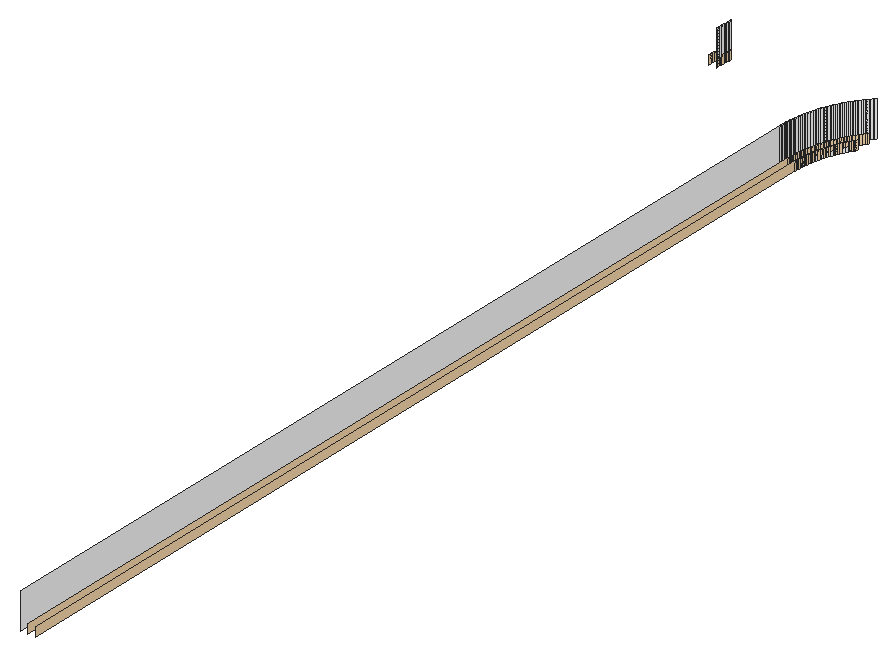
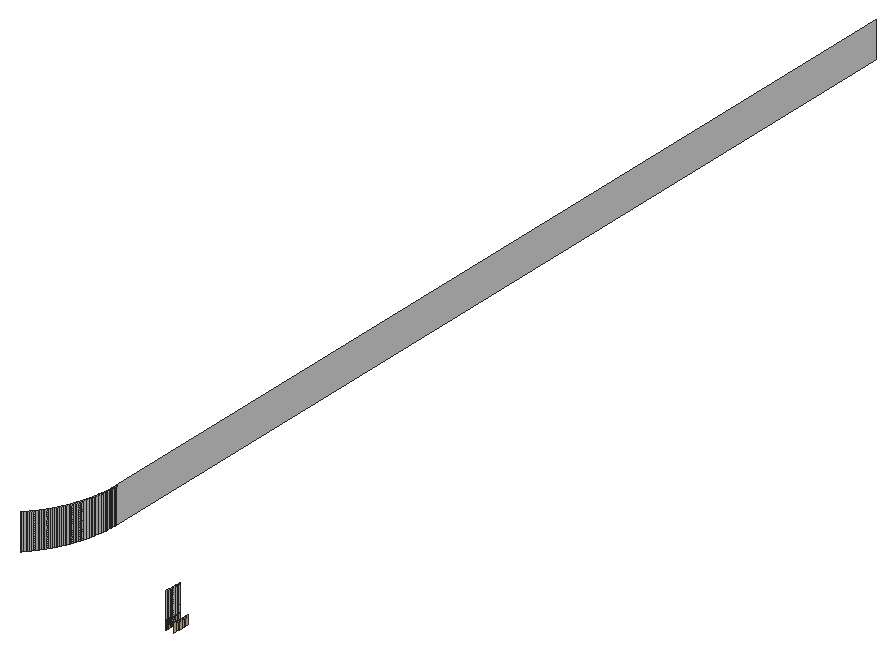
# SketchUp Ruby script. Lengths in inches.
U = 1.inch
M = Sketchup.active_model
def pt(a) = Geom::Point3d.new(a.map { |v| v * U })
def face(e, loops, mat)
  f = e.add_face(loops[0].map { |a| pt(a) })
  loops[1..].each { |l| e.add_face(l.map { |a| pt(a) }).erase! }
  f.material = f.back_material = mat if mat
  f
end
# faces: each face lists its corners as indices into pts; further lists are holes
def faces(e, pts, list, mat = nil) = list.each { |f| face(e, (f[0].is_a?(Array) ? f : [f]).map { |l| l.map { |i| pts[i] } }, mat) }
# xy, xz, yz: faces in a plane at the given z, y or x. An outline is a flat list of corners, or four numbers for a rectangle; further outlines are holes
def ring(l) = l.size == 4 ? [[l[0], l[1]], [l[2], l[1]], [l[2], l[3]], [l[0], l[3]]] : l.each_slice(2).to_a
def flat(e, list, mat, &to3) = list.each { |f| face(e, (f[0].is_a?(Array) ? f : [f]).map { |l| ring(l).map { |u, v| to3.(u, v) } }, mat) }
def xy(e, z, list, mat = nil) = flat(e, list, mat) { |x, y| [x, y, z] }
def xz(e, y, list, mat = nil) = flat(e, list, mat) { |x, z| [x, y, z] }
def yz(e, x, list, mat = nil) = flat(e, list, mat) { |y, z| [x, y, z] }
def lines(e, pts, list) = list.each { |a, b| e.add_line(pt(pts[a]), pt(pts[b])) }
# prism: a flat outline (further loops are holes) pulled along v
def prism(e, loops, v, mat = nil)
  f = face(e, loops, mat); d = Geom::Vector3d.new(v.map { |x| x * U })
  f.pushpull(f.normal.samedirection?(d) ? d.length : -d.length)
end
def box(e, o, s, mat = nil) = prism(e, [[o, [o[0] + s[0], o[1], o[2]], [o[0] + s[0], o[1] + s[1], o[2]], [o[0], o[1] + s[1], o[2]]]], [0, 0, s[2]], mat)
def at(x, y, z, deg = 0) = Geom::Transformation.translation(pt([x, y, z])) * Geom::Transformation.rotation(ORIGIN, Z_AXIS, deg.degrees)
def axes(o, x, y, z) = Geom::Transformation.new([*x, 0, *y, 0, *z, 0, *pt(o).to_a, 1])
def part(name) = M.definitions.add(name)
# library, detail: a bought-in or finely detailed component or shape, given as its bounding box
def library(name, o, s) = part(name).tap { |d| box(d.entities, o, s) }
def detail(e, o, s) = box(e.add_group.entities, o, s)
def put(e, d, t, mat = nil) = e.add_instance(d, t).tap { |i| i.material = mat if mat }
def group(e, t, mat = nil) = e.add_group.tap { |g| g.transformation = t; g.material = mat if mat }.entities
root = M.entities
M.materials.add("False Ceiling Light").color = [254, 223, 179]
M.materials.add("[Quartz Light Grey]").color = [251, 251, 252]
yz(root,22.5,[[216,115.32,216.24,116.49],[216.24,115.32,216.47,116.49]],"False Ceiling Light")
yz(root,23.5,[[215.99,115.32,216.23,116.49],[216.23,115.32,216.45,116.49]],"False Ceiling Light")
yz(root,23.5,[[215.99,115.32,216.23,120],[216.23,115.32,216.45,120]],"[Quartz Light Grey]")
yz(root,41.5,[[78.06,115.32,204.01,120],[204.01,115.32,204.2,120]],"[Quartz Light Grey]")
yz(root,41.51,[[204.41,115.32,204.61,120]],"[Quartz Light Grey]")
yz(root,42.5,[[78.0625,115.32,204.01,116.49],[204.01,115.32,204.19,116.49],[204.19,115.32,204.38,116.49]],"False Ceiling Light")
yz(root,43.5,[[78.0625,115.32,204,116.49],[204,115.32,204.18,116.49],[204.18,115.32,204.35,116.49]],"False Ceiling Light")
yz(root,43.5,[[78.0625,115.32,204,115.91],[204,115.32,204.18,115.91],[204.18,115.32,204.35,115.91]],"[Quartz Light Grey]")
p = [[41.5,204.2,115.32],[41.51,204.41,115.32],[41.51,204.41,120],[41.5,204.2,120],[42.51,204.57,115.32],[42.5,204.38,115.32],
  [42.5,204.38,116.49],[42.51,204.57,116.49],[43.5,204.35,115.32],[43.51,204.53,115.32],[43.51,204.53,116.49],[43.5,204.35,116.49],
  [43.51,204.53,115.32],[43.5,204.35,115.32],[43.5,204.35,115.91],[43.51,204.53,115.91],[43.52,204.71,115.32],[43.52,204.71,116.49],
  [43.52,204.71,115.32],[43.52,204.71,115.91],[41.51,204.61,115.32],[41.52,204.8125,115.32],[41.52,204.8125,120],[41.51,204.61,120],
  [42.52,204.76,115.32],[42.52,204.76,116.49],[43.53,204.88,115.32],[43.53,204.88,116.49],[43.53,204.88,115.32],[43.53,204.88,115.91],
  [41.53,205.01,115.32],[41.53,205.01,120],[42.53,204.95,115.32],[42.53,204.95,116.49],[42.54,205.14,115.32],[42.54,205.14,116.49],
  [43.54,205.06,115.32],[43.54,205.06,116.49],[43.54,205.06,115.32],[43.54,205.06,115.91],[41.55,205.22,115.32],[41.55,205.22,120],
  [42.5625,205.33,115.32],[42.5625,205.33,116.49],[43.56,205.24,115.32],[43.56,205.24,116.49],[43.56,205.24,115.32],[43.56,205.24,115.91],
  [41.56,205.42,115.32],[41.56,205.42,120],[43.57,205.41,115.32],[43.57,205.41,116.49],[43.57,205.41,115.32],[43.57,205.41,115.91],
  [42.58,205.52,115.32],[42.58,205.52,116.49],[41.58,205.62,115.32],[41.58,205.62,120],[43.59,205.59,115.32],[43.59,205.59,116.49],
  [43.59,205.59,115.32],[43.59,205.59,115.91],[42.6,205.7,115.32],[42.6,205.7,116.49],[41.61,205.82,115.32],[41.61,205.82,120],
  [43.62,205.76,115.32],[43.62,205.76,116.49],[43.62,205.76,115.32],[43.62,205.76,115.91],[42.625,205.89,115.32],[42.625,205.89,116.49],
  [41.63,206.02,115.32],[41.63,206.02,120],[43.64,205.9375,115.32],[43.64,205.9375,116.49],[43.64,205.9375,115.32],[43.64,205.9375,115.91],
  [42.65,206.08,115.32],[42.65,206.08,116.49],[43.67,206.11,115.32],[43.67,206.11,116.49],[43.67,206.11,115.32],[43.67,206.11,115.91],
  [41.66,206.22,115.32],[41.66,206.22,120],[42.68,206.27,115.32],[42.68,206.27,116.49],[43.69,206.29,115.32],[43.69,206.29,116.49],
  [43.69,206.29,115.32],[43.69,206.29,115.91],[41.69,206.42,115.32],[41.69,206.42,120],[42.71,206.46,115.32],[42.71,206.46,116.49],
  [43.73,206.46,115.32],[43.73,206.46,116.49],[43.73,206.46,115.32],[43.73,206.46,115.91],[41.72,206.625,115.32],[41.72,206.625,120],
  [42.74,206.64,115.32],[42.74,206.64,116.49],[43.76,206.63,115.32],[43.76,206.63,116.49],[43.76,206.63,115.32],[43.76,206.63,115.91],
  [41.76,206.82,115.32],[41.76,206.82,120],[42.78,206.83,115.32],[42.78,206.83,116.49],[43.79,206.81,115.32],[43.79,206.81,116.49],
  [43.79,206.81,115.32],[43.79,206.81,115.91],[41.8,207.02,115.32],[41.8,207.02,120],[42.82,207.01,115.32],[42.82,207.01,116.49],
  [43.83,206.98,115.32],[43.83,206.98,116.49],[43.83,206.98,115.32],[43.83,206.98,115.91],[41.84,207.22,115.32],[41.84,207.22,120],
  [42.86,207.2,115.32],[42.86,207.2,116.49],[43.87,207.15,115.32],[43.87,207.15,116.49],[43.87,207.15,115.32],[43.87,207.15,115.91],
  [41.88,207.42,115.32],[41.88,207.42,120],[42.9,207.38,115.32],[42.9,207.38,116.49],[43.92,207.32,115.32],[43.92,207.32,116.49],
  [43.92,207.32,115.32],[43.92,207.32,115.91],[43.96,207.49,115.32],[43.96,207.49,116.49],[43.96,207.49,115.32],[43.96,207.49,115.91],
  [41.93,207.62,115.32],[41.93,207.62,120],[42.95,207.57,115.32],[42.95,207.57,116.49],[44.01,207.66,115.32],[44.01,207.66,116.49],
  [44.01,207.66,115.32],[44.01,207.66,115.91],[41.98,207.82,115.32],[41.98,207.82,120],[42.99,207.75,115.32],[42.99,207.75,116.49],
  [44.06,207.83,115.32],[44.06,207.83,116.49],[44.06,207.83,115.32],[44.06,207.83,115.91],[42.03,208.01,115.32],[42.03,208.01,120],
  [43.04,207.9375,115.32],[43.04,207.9375,116.49],[44.11,208,115.32],[44.11,208,116.49],[44.11,208,115.32],[44.11,208,115.91],
  [43.1,208.12,115.32],[43.1,208.12,116.49],[42.08,208.21,115.32],[42.08,208.21,120],[44.16,208.17,115.32],[44.16,208.17,116.49],
  [44.16,208.17,115.32],[44.16,208.17,115.91],[43.15,208.3,115.32],[43.15,208.3,116.49],[42.14,208.4,115.32],[42.14,208.4,120],
  [44.22,208.34,115.32],[44.22,208.34,116.49],[44.22,208.34,115.32],[44.22,208.34,115.91],[43.21,208.48,115.32],[43.21,208.48,116.49],
  [44.27,208.51,115.32],[44.27,208.51,116.49],[44.27,208.51,115.32],[44.27,208.51,115.91],[42.2,208.6,115.32],[42.2,208.6,120],
  [43.27,208.66,115.32],[43.27,208.66,116.49],[44.33,208.67,115.32],[44.33,208.67,116.49],[44.33,208.67,115.32],[44.33,208.67,115.91],
  [42.26,208.79,115.32],[42.26,208.79,120],[43.33,208.84,115.32],[43.33,208.84,116.49],[44.4,208.84,115.32],[44.4,208.84,116.49],
  [44.4,208.84,115.32],[44.4,208.84,115.91],[42.32,208.98,115.32],[42.32,208.98,120],[43.4,209.02,115.32],[43.4,209.02,116.49],
  [44.46,209,115.32],[44.46,209,116.49],[44.46,209,115.32],[44.46,209,115.91],[42.39,209.17,115.32],[42.39,209.17,120],
  [43.46,209.2,115.32],[43.46,209.2,116.49],[44.53,209.17,115.32],[44.53,209.17,116.49],[44.53,209.17,115.32],[44.53,209.17,115.91],
  [42.46,209.36,115.32],[42.46,209.36,120],[43.53,209.375,115.32],[43.53,209.375,116.49],[44.6,209.33,115.32],[44.6,209.33,116.49],
  [44.6,209.33,115.32],[44.6,209.33,115.91],[44.67,209.49,115.32],[44.67,209.49,116.49],[44.67,209.49,115.32],[44.67,209.49,115.91],
  [42.53,209.55,115.32],[42.53,209.55,120],[43.6,209.55,115.32],[43.6,209.55,116.49],[43.68,209.72,115.32],[43.68,209.72,116.49],
  [44.74,209.65,115.32],[44.74,209.65,116.49],[44.74,209.65,115.32],[44.74,209.65,115.91],[42.6,209.74,115.32],[42.6,209.74,120],
  [42.68,209.93,115.32],[42.68,209.93,120],[43.75,209.9,115.32],[43.75,209.9,116.49],[44.82,209.8125,115.32],[44.82,209.8125,116.49],
  [44.82,209.8125,115.32],[44.82,209.8125,115.91],[44.89,209.97,115.32],[44.89,209.97,116.49],[44.89,209.97,115.32],[44.89,209.97,115.91],
  [42.76,210.12,115.32],[42.76,210.12,120],[43.83,210.07,115.32],[43.83,210.07,116.49],[44.97,210.13,115.32],[44.97,210.13,116.49],
  [44.97,210.13,115.32],[44.97,210.13,115.91],[42.84,210.3,115.32],[42.84,210.3,120],[43.91,210.24,115.32],[43.91,210.24,116.49],
  [45.05,210.29,115.32],[45.05,210.29,116.49],[45.05,210.29,115.32],[45.05,210.29,115.91],[44,210.41,115.32],[44,210.41,116.49],
  [42.92,210.49,115.32],[42.92,210.49,120],[45.14,210.44,115.32],[45.14,210.44,116.49],[45.14,210.44,115.32],[45.14,210.44,115.91],
  [44.08,210.58,115.32],[44.08,210.58,116.49],[45.22,210.6,115.32],[45.22,210.6,116.49],[45.22,210.6,115.32],[45.22,210.6,115.91],
  [43.01,210.67,115.32],[43.01,210.67,120],[44.17,210.75,115.32],[44.17,210.75,116.49],[45.31,210.75,115.32],[45.31,210.75,116.49],
  [45.31,210.75,115.32],[45.31,210.75,115.91],[43.1,210.86,115.32],[43.1,210.86,120],[44.26,210.92,115.32],[44.26,210.92,116.49],
  [45.4,210.9,115.32],[45.4,210.9,116.49],[45.4,210.9,115.32],[45.4,210.9,115.91],[43.1875,211.04,115.32],[43.1875,211.04,120],
  [44.35,211.09,115.32],[44.35,211.09,116.49],[45.49,211.05,115.32],[45.49,211.05,116.49],[45.49,211.05,115.32],[45.49,211.05,115.91],
  [43.28,211.22,115.32],[43.28,211.22,120],[44.44,211.25,115.32],[44.44,211.25,116.49],[45.58,211.2,115.32],[45.58,211.2,116.49],
  [45.58,211.2,115.32],[45.58,211.2,115.91],[43.38,211.4,115.32],[43.38,211.4,120],[45.68,211.35,115.32],[45.68,211.35,116.49],
  [45.68,211.35,115.32],[45.68,211.35,115.91],[44.54,211.41,115.32],[44.54,211.41,116.49],[43.48,211.57,115.32],[43.48,211.57,120],
  [44.64,211.58,115.32],[44.64,211.58,116.49],[45.78,211.5,115.32],[45.78,211.5,116.49],[45.78,211.5,115.32],[45.78,211.5,115.91],
  [43.58,211.75,115.32],[43.58,211.75,120],[44.74,211.74,115.32],[44.74,211.74,116.49],[44.84,211.9,115.32],[44.84,211.9,116.49],
  [43.68,211.93,115.32],[43.68,211.93,120],[43.78,212.1,115.32],[43.78,212.1,120],[44.94,212.06,115.32],[44.94,212.06,116.49],
  [43.89,212.27,115.32],[43.89,212.27,120],[45.05,212.21,115.32],[45.05,212.21,116.49],[45.16,212.37,115.32],[45.16,212.37,116.49],
  [44,212.44,115.32],[44,212.44,120],[44.11,212.61,115.32],[44.11,212.61,120],[45.27,212.52,115.32],[45.27,212.52,116.49],
  [45.38,212.68,115.32],[45.38,212.68,116.49],[44.23,212.78,115.32],[44.23,212.78,120],[45.5,212.83,115.32],[45.5,212.83,116.49],
  [44.34,212.95,115.32],[44.34,212.95,120],[45.61,212.98,115.32],[45.61,212.98,116.49],[44.46,213.11,115.32],[44.46,213.11,120],
  [45.73,213.125,115.32],[45.73,213.125,116.49],[44.58,213.27,115.32],[44.58,213.27,120],[45.85,213.27,115.32],[45.85,213.27,116.49],
  [44.7,213.4375,115.32],[44.7,213.4375,120],[44.83,213.6,115.32],[44.83,213.6,120],[44.95,213.75,115.32],[44.95,213.75,120],
  [45.08,213.91,115.32],[45.08,213.91,120],[45.21,214.07,115.32],[45.21,214.07,120],[45.35,214.22,115.32],[45.35,214.22,120],
  [45.48,214.37,115.32],[45.48,214.37,120],[45.62,214.52,115.32],[45.62,214.52,120],[45.76,214.67,115.32],[45.76,214.67,120],
  [22.51,216.71,115.32],[22.5,216.47,115.32],[22.5,216.47,116.49],[22.51,216.71,116.49],[23.51,216.68,115.32],[23.5,216.45,115.32],
  [23.5,216.45,120],[23.51,216.68,120],[23.5,216.45,115.32],[23.51,216.68,115.32],[23.51,216.68,116.49],[23.5,216.45,116.49],
  [22.52,216.94,115.32],[22.52,216.94,116.49],[23.52,216.9,115.32],[23.52,216.9,120],[23.52,216.9,115.32],[23.52,216.9,116.49],
  [22.53,217.18,115.32],[22.53,217.18,116.49],[23.53,217.125,115.32],[23.53,217.125,120],[23.53,217.125,115.32],[23.53,217.125,116.49],
  [23.54,217.35,115.32],[23.54,217.35,120],[23.54,217.35,115.32],[23.54,217.35,116.49],[22.54,217.41,115.32],[22.54,217.41,116.49],
  [23.56,217.57,115.32],[23.56,217.57,120],[23.56,217.57,115.32],[23.56,217.57,116.49],[22.56,217.65,115.32],[22.56,217.65,116.49],
  [22.58,217.88,115.32],[22.58,217.88,116.49],[23.58,217.8,115.32],[23.58,217.8,120],[23.58,217.8,115.32],[23.58,217.8,116.49],
  [23.6,218.02,115.32],[23.6,218.02,120],[23.6,218.02,115.32],[23.6,218.02,116.49],[22.6,218.12,115.32],[22.6,218.12,116.49],
  [23.62,218.25,115.32],[23.62,218.25,120],[23.62,218.25,115.32],[23.62,218.25,116.49],[45,215.9375,120],[45,216,120],
  [45.0625,216,120]]
faces(root,p,[[0,1,2,3],[12,13,14,15],[18,12,15,19],[20,21,22,23],[28,18,19,29],[21,30,31,22],[38,28,29,39],[30,40,41,31],
  [46,38,39,47],[40,48,49,41],[52,46,47,53],[48,56,57,49],[60,52,53,61],[56,64,65,57],[68,60,61,69],[64,72,73,65],
  [76,68,69,77],[82,76,77,83],[72,84,85,73],[90,82,83,91],[84,92,93,85],[98,90,91,99],[92,100,101,93],[106,98,99,107],
  [100,108,109,101],[114,106,107,115],[108,116,117,109],[122,114,115,123],[116,124,125,117],[130,122,123,131],[124,132,133,125],[138,130,131,139],
  [142,138,139,143],[132,144,145,133],[150,142,143,151],[144,152,153,145],[158,150,151,159],[152,160,161,153],[166,158,159,167],[160,170,171,161],
  [174,166,167,175],[170,178,179,171],[182,174,175,183],[188,182,183,189],[178,190,191,179],[196,188,189,197],[190,198,199,191],[204,196,197,205],
  [198,206,207,199],[212,204,205,213],[206,214,215,207],[220,212,213,221],[214,222,223,215],[228,220,221,229],[232,228,229,233],[222,234,235,223],
  [242,232,233,243],[234,244,245,235],[244,246,247,245],[252,242,243,253],[256,252,253,257],[246,258,259,247],[264,256,257,265],[258,266,267,259],
  [272,264,265,273],[266,276,277,267],[280,272,273,281],[286,280,281,287],[276,288,289,277],[294,286,287,295],[288,296,297,289],[302,294,295,303],
  [296,304,305,297],[310,302,303,311],[304,312,313,305],[318,310,311,319],[312,320,321,313],[324,318,319,325],[320,328,329,321],[334,324,325,335],
  [328,336,337,329],[336,342,343,337],[342,344,345,343],[344,348,349,345],[348,354,355,349],[354,356,357,355],[356,362,363,357],[362,366,367,363],
  [366,370,371,367],[370,374,375,371],[374,378,379,375],[378,380,381,379],[380,382,383,381],[382,384,385,383],[384,386,387,385],[386,388,389,387],
  [388,390,391,389],[390,392,393,391],[392,394,395,393],[400,401,402,403],[410,400,403,411],[416,410,411,417],[420,416,417,421],[426,420,421,427],
  [434,426,427,435],[438,434,435,439],[444,438,439,445]],"[Quartz Light Grey]")
faces(root,p,[[4,5,6,7],[8,9,10,11],[9,16,17,10],[24,4,7,25],[16,26,27,17],[32,24,25,33],[34,32,33,35],[26,36,37,27],
  [42,34,35,43],[36,44,45,37],[44,50,51,45],[54,42,43,55],[50,58,59,51],[62,54,55,63],[58,66,67,59],[70,62,63,71],
  [66,74,75,67],[78,70,71,79],[74,80,81,75],[86,78,79,87],[80,88,89,81],[94,86,87,95],[88,96,97,89],[102,94,95,103],
  [96,104,105,97],[110,102,103,111],[104,112,113,105],[118,110,111,119],[112,120,121,113],[126,118,119,127],[120,128,129,121],[134,126,127,135],
  [128,136,137,129],[136,140,141,137],[146,134,135,147],[140,148,149,141],[154,146,147,155],[148,156,157,149],[162,154,155,163],[156,164,165,157],
  [168,162,163,169],[164,172,173,165],[176,168,169,177],[172,180,181,173],[184,176,177,185],[180,186,187,181],[192,184,185,193],[186,194,195,187],
  [200,192,193,201],[194,202,203,195],[208,200,201,209],[202,210,211,203],[216,208,209,217],[210,218,219,211],[224,216,217,225],[218,226,227,219],
  [226,230,231,227],[236,224,225,237],[238,236,237,239],[230,240,241,231],[248,238,239,249],[240,250,251,241],[250,254,255,251],[260,248,249,261],
  [254,262,263,255],[268,260,261,269],[262,270,271,263],[274,268,269,275],[270,278,279,271],[282,274,275,283],[278,284,285,279],[290,282,283,291],
  [284,292,293,285],[298,290,291,299],[292,300,301,293],[306,298,299,307],[300,308,309,301],[314,306,307,315],[308,316,317,309],[316,322,323,317],
  [326,314,315,327],[330,326,327,331],[322,332,333,323],[338,330,331,339],[340,338,339,341],[346,340,341,347],[350,346,347,351],[352,350,351,353],
  [358,352,353,359],[360,358,359,361],[364,360,361,365],[368,364,365,369],[372,368,369,373],[376,372,373,377],[396,397,398,399],[404,405,406,407],
  [408,396,399,409],[405,412,413,406],[414,408,409,415],[412,418,419,413],[418,422,423,419],[424,414,415,425],[422,428,429,423],[430,424,425,431],
  [432,430,431,433],[428,436,437,429],[436,440,441,437],[442,432,433,443],[440,446,447,441]],"False Ceiling Light")
lines(root,p,[[448,449],[449,450]])
